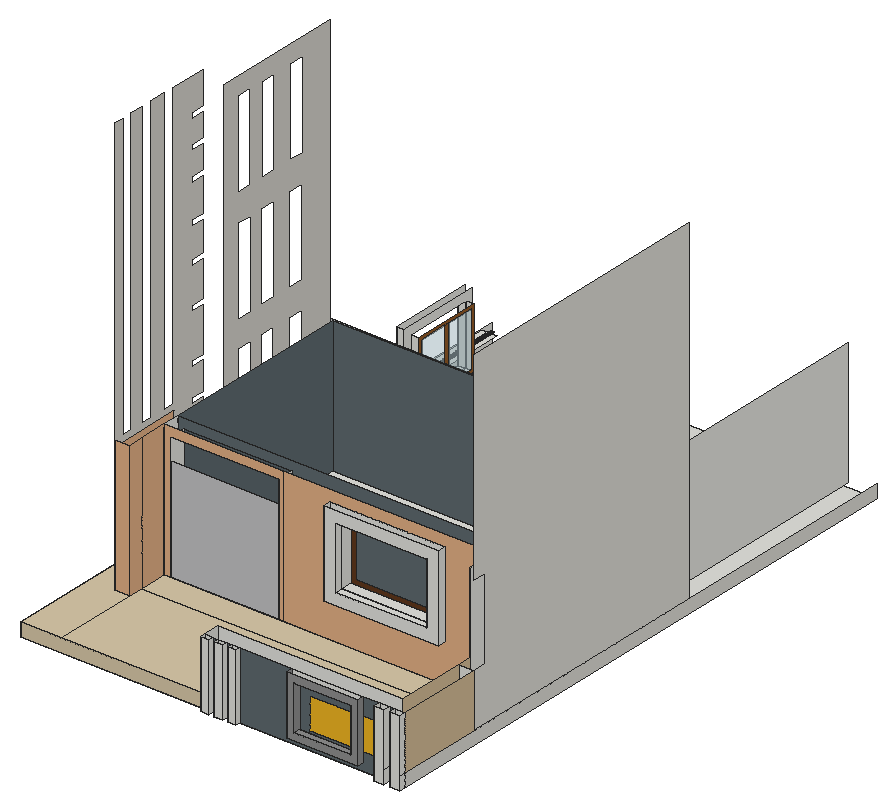
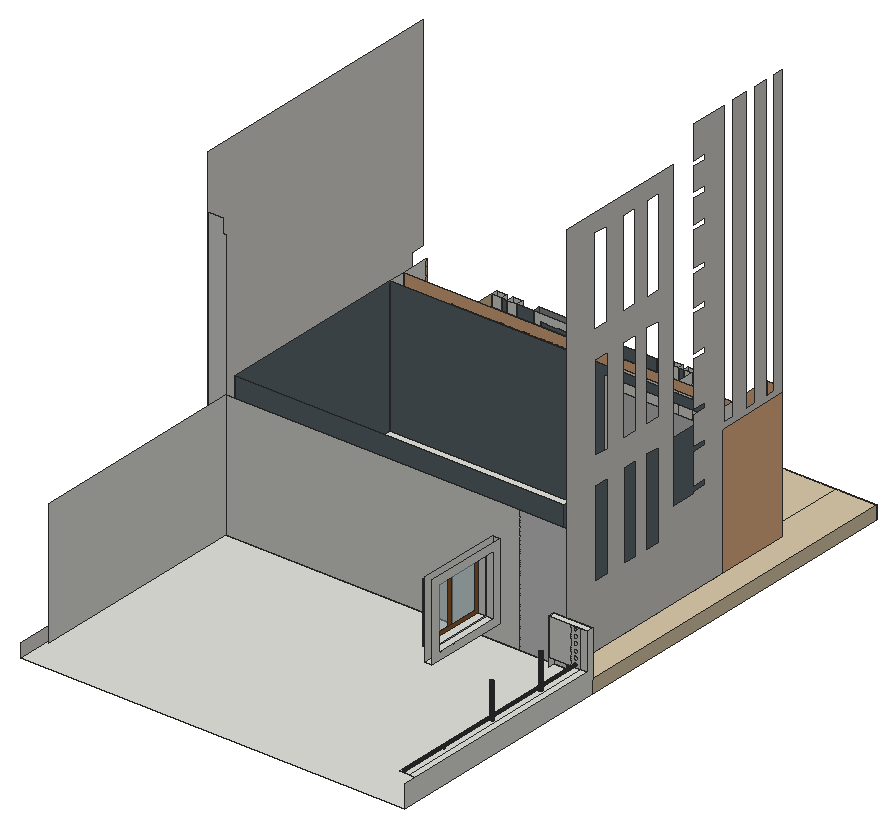
# SketchUp Ruby script. Lengths in inches.
U = 1.inch
M = Sketchup.active_model
def pt(a) = Geom::Point3d.new(a.map { |v| v * U })
def face(e, loops, mat)
  f = e.add_face(loops[0].map { |a| pt(a) })
  loops[1..].each { |l| e.add_face(l.map { |a| pt(a) }).erase! }
  f.material = f.back_material = mat if mat
  f
end
# faces: each face lists its corners as indices into pts; further lists are holes
def faces(e, pts, list, mat = nil) = list.each { |f| face(e, (f[0].is_a?(Array) ? f : [f]).map { |l| l.map { |i| pts[i] } }, mat) }
# xy, xz, yz: faces in a plane at the given z, y or x. An outline is a flat list of corners, or four numbers for a rectangle; further outlines are holes
def ring(l) = l.size == 4 ? [[l[0], l[1]], [l[2], l[1]], [l[2], l[3]], [l[0], l[3]]] : l.each_slice(2).to_a
def flat(e, list, mat, &to3) = list.each { |f| face(e, (f[0].is_a?(Array) ? f : [f]).map { |l| ring(l).map { |u, v| to3.(u, v) } }, mat) }
def xy(e, z, list, mat = nil) = flat(e, list, mat) { |x, y| [x, y, z] }
def xz(e, y, list, mat = nil) = flat(e, list, mat) { |x, z| [x, y, z] }
def yz(e, x, list, mat = nil) = flat(e, list, mat) { |y, z| [x, y, z] }
def lines(e, pts, list) = list.each { |a, b| e.add_line(pt(pts[a]), pt(pts[b])) }
# prism: a flat outline (further loops are holes) pulled along v
def prism(e, loops, v, mat = nil)
  f = face(e, loops, mat); d = Geom::Vector3d.new(v.map { |x| x * U })
  f.pushpull(f.normal.samedirection?(d) ? d.length : -d.length)
end
def box(e, o, s, mat = nil) = prism(e, [[o, [o[0] + s[0], o[1], o[2]], [o[0] + s[0], o[1] + s[1], o[2]], [o[0], o[1] + s[1], o[2]]]], [0, 0, s[2]], mat)
def at(x, y, z, deg = 0) = Geom::Transformation.translation(pt([x, y, z])) * Geom::Transformation.rotation(ORIGIN, Z_AXIS, deg.degrees)
def axes(o, x, y, z) = Geom::Transformation.new([*x, 0, *y, 0, *z, 0, *pt(o).to_a, 1])
def part(name) = M.definitions.add(name)
# library, detail: a bought-in or finely detailed component or shape, given as its bounding box
def library(name, o, s) = part(name).tap { |d| box(d.entities, o, s) }
def detail(e, o, s) = box(e.add_group.entities, o, s)
def put(e, d, t, mat = nil) = e.add_instance(d, t).tap { |i| i.material = mat if mat }
def group(e, t, mat = nil) = e.add_group.tap { |g| g.transformation = t; g.material = mat if mat }.entities
root = M.entities
M.materials.add("[0045_Goldenrod]").color = [239, 181, 35]
M.materials.add("[Blinds Vertical Pattern]").color = [212, 212, 214]
M.materials.add("[Cladding Siding Tan]").color = [226, 176, 133]
M.materials.add("[Color M04]").color = [142, 142, 142]
M.materials.add("[Color M07]").color = [58, 58, 58]
M.materials.add("[Fencing Metal Straight]").color = [194, 195, 196]
M.materials.add("[Field Square Tile]").color = [217, 201, 169]
M.materials.add("[Formica Beige]").color = [211, 187, 149]
M.materials.add("[Formica Speckled Grey]").color = [94, 105, 111]
M.materials.add("[Terrazzo Tile Light]").color = [219, 217, 210]
M.materials.add("[Tile Travertine 2 inch]").color = [211, 208, 201]
M.materials.add("[Translucent Glass Safety]").color = [204, 235, 244]
M.materials["[Translucent Glass Safety]"].alpha = 0.5
M.materials.add("[Wood Floor Parquet]").color = [145, 89, 39]
M.materials.add("[Wood Veneer 01]").color = [96, 56, 29]
xy(root,0,[[499.38,0,512.5625,9.1875],[520.19,0,533.375,9.1875],[265.43,2.6875,276.6,9.1875],[283.37,2.6875,294.54,9.1875],[301.06,2.6875,312.23,9.1875],
  [18.625,9.1875,533.375,797.6875]])
xy(root,10.4375,[[382.41,0,477.59,9.1875]],"[Color M04]")
xy(root,18,[[53.375,123.625,53.375,483.625,533.375,483.625,533.375,123.625,513.45,123.625,513.45,463.7,73.3,463.7,73.3,123.625],[73.3,181.59,81.47,204.11],[81.47,181.59,226.34,204.11],[226.34,181.59,513.45,204.11],[73.3,204.11,513.45,463.7]])
xy(root,18,[[18.625,9.1875,73.3,9.1875,73.3,123.625,53.375,123.625,53.375,483.625,18.625,483.625],[73.3,9.1875,265.43,9.1875,265.43,31.125,513.45,31.125,513.45,143.55,73.3,143.55],[73.3,143.55,513.45,181.59]],"[Field Square Tile]")
xy(root,20.19,[[392.16,0,467.84,9.1875]],"[Color M04]")
xy(root,29.4375,[[18.625,492.63,26.76,779.875],[[26.76,492.63,40.07,779.875],[32.79,632.33,32.19,632.41,31.63,632.64,31.15,633.01,30.79,633.49,30.56,634.04,30.48,634.64,30.56,635.24,30.79,635.8,31.15,636.28,31.63,636.65,32.19,636.875,32.79,636.96,33.39,636.875,33.95,636.65,34.42,636.28,34.79,635.8,35.02,635.24,35.1,634.64,35.02,634.04,34.79,633.49,34.42,633.01,33.95,632.64,33.39,632.41],[32.79,550.08,32.19,550.16,31.63,550.39,31.15,550.76,30.79,551.24,30.56,551.79,30.48,552.39,30.56,552.99,30.79,553.55,31.15,554.03,31.63,554.4,32.19,554.625,32.79,554.71,33.39,554.625,33.95,554.4,34.42,554.03,34.79,553.55,35.02,552.99,35.1,552.39,35.02,551.79,34.79,551.24,34.42,550.76,33.95,550.39,33.39,550.16],[32.79,711.89,32.19,711.97,31.63,712.2,31.15,712.57,30.79,713.05,30.56,713.61,30.48,714.21,30.56,714.8,30.79,715.36,31.15,715.84,31.63,716.21,32.19,716.4375,32.79,716.52,33.39,716.4375,33.95,716.21,34.42,715.84,34.79,715.36,35.02,714.8,35.1,714.21,35.02,713.61,34.79,713.05,34.42,712.57,33.95,712.2,33.39,711.97]],[32.79,550.08,32.19,550.16,31.63,550.39,31.15,550.76,30.79,551.24,30.56,551.79,30.48,552.39,30.56,552.99,30.79,553.55,31.15,554.03,31.63,554.4,32.19,554.625,32.79,554.71,33.39,554.625,33.95,554.4,34.42,554.03,34.79,553.55,35.02,552.99,35.1,552.39,35.02,551.79,34.79,551.24,34.42,550.76,33.95,550.39,33.39,550.16],[32.79,632.33,32.19,632.41,31.63,632.64,31.15,633.01,30.79,633.49,30.56,634.04,30.48,634.64,30.56,635.24,30.79,635.8,31.15,636.28,31.63,636.65,32.19,636.875,32.79,636.96,33.39,636.875,33.95,636.65,34.42,636.28,34.79,635.8,35.02,635.24,35.1,634.64,35.02,634.04,34.79,633.49,34.42,633.01,33.95,632.64,33.39,632.41]])
xy(root,68.97,[[295.4375,171.21,449,181.59]])
xy(root,72.6,[[106.94,528.53,116.75,641.54]])
xy(root,75.3125,[[32.79,550.08,33.39,550.16,33.95,550.39,34.42,550.76,34.79,551.24,35.02,551.79,35.1,552.39,35.02,552.99,34.79,553.55,34.42,554.03,33.95,554.4,33.39,554.625,32.79,554.71,32.19,554.625,31.63,554.4,31.15,554.03,30.79,553.55,30.56,552.99,30.48,552.39,30.56,551.79,30.79,551.24,31.15,550.76,31.63,550.39,32.19,550.16]],"[Color M07]")
xy(root,76.375,[[32.79,632.33,33.39,632.41,33.95,632.64,34.42,633.01,34.79,633.49,35.02,634.04,35.1,634.64,35.02,635.24,34.79,635.8,34.42,636.28,33.95,636.65,33.39,636.875,32.79,636.96,32.19,636.875,31.63,636.65,31.15,636.28,30.79,635.8,30.56,635.24,30.48,634.64,30.56,634.04,30.79,633.49,31.15,633.01,31.63,632.64,32.19,632.41]],"[Color M07]")
xy(root,78.6875,[[18.625,483.625,70.21,492.63]])
xy(root,79.81,[[392.16,0,467.84,9.1875]])
xy(root,83.1,[[106.94,539.02,116.75,631.05],[116.75,539.02,128.38,631.05]])
xy(root,84.57,[[311.03,171.21,433.4,181.59],[311.03,181.59,433.4,197.15]])
xz(root,0,[[499.38,0,512.5625,89.5625],[520.19,0,533.375,89.5625]])
xz(root,0,[[[382.41,10.4375,477.59,89.5625],[392.16,20.19,467.84,79.81]]],"[Color M04]")
xz(root,2.6875,[[265.43,0,276.6,89.5625],[283.37,0,294.54,89.5625],[301.06,0,312.23,89.5625]])
xz(root,9.1875,[[265.43,0,276.6,89.5625],[283.37,0,294.54,89.5625],[301.06,0,312.23,89.5625],[499.38,0,512.5625,89.5625],[520.19,0,533.375,89.5625],
  [[382.41,10.4375,477.59,89.5625],[392.16,20.19,467.84,79.81]]])
xz(root,9.1875,[[406.65,23.29,467.84,65.73],[477.59,23.29,499.38,65.73]],"[0045_Goldenrod]")
xz(root,9.1875,[[18.625,0,265.43,18]],"[Field Square Tile]")
xz(root,9.1875,[[276.6,0,283.37,89.5625],[294.54,0,301.06,89.5625],[312.23,0,499.38,0,499.38,23.29,477.59,23.29,477.59,10.4375,382.41,10.4375,382.41,89.5625,312.23,89.5625],[512.5625,0,520.19,89.5625],[392.16,20.19,467.84,20.19,467.84,23.29,406.65,23.29,406.65,65.73,467.84,65.73,467.84,79.81,392.16,79.81],
  [477.59,65.73,499.38,89.5625]],"[Formica Speckled Grey]")
xz(root,31.125,[[265.43,18,513.45,89.5625]])
xz(root,123.625,[[513.45,18,533.375,89.5625]])
xz(root,123.625,[[53.375,18,73.3,198]],"[Cladding Siding Tan]")
xz(root,171.21,[[[295.4375,68.97,449,183.35],[311.03,84.57,433.4,167.75]]])
xz(root,181.59,[[[295.4375,68.97,449,183.35],[311.03,84.57,433.4,167.75]]])
xz(root,181.59,[[73.3,18,81.47,18,81.47,186,226.34,186,226.34,18,231.56,18,231.56,198,73.3,198],[[231.56,18,513.45,198],[295.4375,68.97,449,183.35]]],"[Cladding Siding Tan]")
xz(root,181.59,[[81.47,18,226.34,156.98]],"[Fencing Metal Straight]")
xz(root,197.15,[[[311.03,84.57,433.4,167.75],[316.66,90.2,427.78,162.125]]],"[Wood Veneer 01]")
xz(root,204.11,[[73.3,18,73.3,198,513.45,198,513.45,18,226.34,18,226.34,186,81.47,186,81.47,18]],"[Formica Speckled Grey]")
xz(root,463.7,[[73.3,18,513.45,198]],"[Formica Speckled Grey]")
xz(root,483.625,[[18.625,18,53.375,78.6875],[53.375,18,70.21,78.6875],[116.75,18,509.21,185.6875],[509.21,18,509.21,378,513.45,378,513.45,396.875,533.375,396.875,533.375,18]])
xz(root,483.625,[[70.21,18,70.21,78.6875,53.375,78.6875,53.375,185.6875,116.75,185.6875,116.75,18]],"[Blinds Vertical Pattern]")
xz(root,492.63,[[18.625,29.4375,26.76,78.6875],[[26.76,29.4375,40.07,78.6875],[34.16,73.8,34.63,73.87,35.07,74.05,35.44,74.34,35.73,74.71,35.91,75.15,35.97,75.62,35.91,76.09,35.73,76.52,35.44,76.9,35.07,77.1875,34.63,77.37,34.16,77.43,33.69,77.37,33.25,77.1875,32.88,76.9,32.59,76.52,32.41,76.09,32.35,75.62,32.41,75.15,32.59,74.71,32.88,74.34,33.25,74.05,33.69,73.87],[34.16,39.43,34.63,39.49,35.07,39.67,35.44,39.96,35.73,40.34,35.91,40.77,35.97,41.24,35.91,41.71,35.73,42.15,35.44,42.52,35.07,42.8125,34.63,42.99,34.16,43.05,33.69,42.99,33.25,42.8125,32.88,42.52,32.59,42.15,32.41,41.71,32.35,41.24,32.41,40.77,32.59,40.34,32.88,39.96,33.25,39.67,33.69,39.49],[34.16,65.12,34.63,65.18,35.07,65.36,35.44,65.65,35.73,66.02,35.91,66.46,35.97,66.93,35.91,67.4,35.73,67.84,35.44,68.21,35.07,68.5,34.63,68.68,34.16,68.74,33.69,68.68,33.25,68.5,32.88,68.21,32.59,67.84,32.41,67.4,32.35,66.93,32.41,66.46,32.59,66.02,32.88,65.65,33.25,65.36,33.69,65.18],[34.16,47.68,34.63,47.74,35.07,47.92,35.44,48.21,35.73,48.59,35.91,49.02,35.97,49.49,35.91,49.96,35.73,50.4,35.44,50.77,35.07,51.0625,34.63,51.24,34.16,51.3,33.69,51.24,33.25,51.0625,32.88,50.77,32.59,50.4,32.41,49.96,32.35,49.49,32.41,49.02,32.59,48.59,32.88,48.21,33.25,47.92,33.69,47.74],[34.16,56.74,34.63,56.8,35.07,56.99,35.44,57.27,35.73,57.65,35.91,58.09,35.97,58.55,35.91,59.02,35.73,59.46,35.44,59.84,35.07,60.125,34.63,60.31,34.16,60.37,33.69,60.31,33.25,60.125,32.88,59.84,32.59,59.46,32.41,59.02,32.35,58.55,32.41,58.09,32.59,57.65,32.88,57.27,33.25,56.99,33.69,56.8],[34.16,31.24,34.63,31.3,35.07,31.49,35.44,31.77,35.73,32.15,35.91,32.59,35.97,33.05,35.91,33.52,35.73,33.96,35.44,34.34,35.07,34.625,34.63,34.81,34.16,34.87,33.69,34.81,33.25,34.625,32.88,34.34,32.59,33.96,32.41,33.52,32.35,33.05,32.41,32.59,32.59,32.15,32.88,31.77,33.25,31.49,33.69,31.3]],[40.07,29.4375,70.21,78.6875],[34.16,31.24,34.63,31.3,35.07,31.49,35.44,31.77,35.73,32.15,35.91,32.59,35.97,33.05,35.91,33.52,35.73,33.96,35.44,34.34,35.07,34.625,34.63,34.81,34.16,34.87,33.69,34.81,33.25,34.625,32.88,34.34,32.59,33.96,32.41,33.52,32.35,33.05,32.41,32.59,32.59,32.15,32.88,31.77,33.25,31.49,33.69,31.3],[34.16,39.43,34.63,39.49,35.07,39.67,35.44,39.96,35.73,40.34,35.91,40.77,35.97,41.24,35.91,41.71,35.73,42.15,35.44,42.52,35.07,42.8125,34.63,42.99,34.16,43.05,33.69,42.99,33.25,42.8125,32.88,42.52,32.59,42.15,32.41,41.71,32.35,41.24,32.41,40.77,32.59,40.34,32.88,39.96,33.25,39.67,33.69,39.49],
  [34.16,47.68,34.63,47.74,35.07,47.92,35.44,48.21,35.73,48.59,35.91,49.02,35.97,49.49,35.91,49.96,35.73,50.4,35.44,50.77,35.07,51.0625,34.63,51.24,34.16,51.3,33.69,51.24,33.25,51.0625,32.88,50.77,32.59,50.4,32.41,49.96,32.35,49.49,32.41,49.02,32.59,48.59,32.88,48.21,33.25,47.92,33.69,47.74],[34.16,56.74,34.63,56.8,35.07,56.99,35.44,57.27,35.73,57.65,35.91,58.09,35.97,58.55,35.91,59.02,35.73,59.46,35.44,59.84,35.07,60.125,34.63,60.31,34.16,60.37,33.69,60.31,33.25,60.125,32.88,59.84,32.59,59.46,32.41,59.02,32.35,58.55,32.41,58.09,32.59,57.65,32.88,57.27,33.25,56.99,33.69,56.8],[34.16,65.12,34.63,65.18,35.07,65.36,35.44,65.65,35.73,66.02,35.91,66.46,35.97,66.93,35.91,67.4,35.73,67.84,35.44,68.21,35.07,68.5,34.63,68.68,34.16,68.74,33.69,68.68,33.25,68.5,32.88,68.21,32.59,67.84,32.41,67.4,32.35,66.93,32.41,66.46,32.59,66.02,32.88,65.65,33.25,65.36,33.69,65.18],[34.16,73.8,34.63,73.87,35.07,74.05,35.44,74.34,35.73,74.71,35.91,75.15,35.97,75.62,35.91,76.09,35.73,76.52,35.44,76.9,35.07,77.1875,34.63,77.37,34.16,77.43,33.69,77.37,33.25,77.1875,32.88,76.9,32.59,76.52,32.41,76.09,32.35,75.62,32.41,75.15,32.59,74.71,32.88,74.34,33.25,74.05,33.69,73.87]])
xz(root,528.53,[[106.94,72.6,116.75,174.66]])
xz(root,539.02,[[106.94,83.1,116.75,164.17],[116.75,83.1,128.38,164.17]])
xz(root,631.05,[[106.94,83.1,116.75,164.17],[116.75,83.1,128.38,164.17]])
yz(root,18.625,[[483.625,0,483.625,78.6875,492.63,78.6875,492.63,29.4375,797.6875,29.4375,797.6875,0]])
yz(root,18.625,[[9.1875,0,483.625,18]],"[Field Square Tile]")
yz(root,53.375,[[123.625,18,222.87,189.9375]],"[Cladding Siding Tan]")
yz(root,53.375,[[[222.87,18,222.87,189.9375,123.625,189.9375,123.625,577.3125,136.75,577.3125,136.75,198,151.32,198,151.32,577.3125,169.81,577.3125,169.81,198,184.38,198,184.38,577.3125,206.12,577.3125,206.12,198,220.7,198,220.7,577.3125,270.46,577.3125,270.46,533.22,253.03,533.22,253.03,526.41,270.46,526.41,270.46,495.16,253.03,495.16,253.03,488.34,270.46,488.34,270.46,456.47,253.03,456.47,253.03,449.66,270.46,449.66,270.46,404.47,253.03,404.47,253.03,397.66,270.46,397.66,270.46,356.97,253.03,356.97,253.03,350.16,270.46,350.16,270.46,301.97,253.03,301.97,253.03,295.16,270.46,295.16,270.46,235.53,253.03,235.53,253.03,228.72,270.46,228.72,270.46,191.16,253.03,191.16,253.03,184.34,270.46,184.34,270.46,143.41,253.03,143.41,253.03,136.59,270.46,136.59,270.46,134.2,306.125,134.2,306.125,543.2,483.625,543.2,483.625,18],[417,404.29,438.25,519.67],[415.62,251.86,436.87,367.23],[415.12,101.04,436.37,216.42],[369.37,404.29,390.62,519.67],[329.18,404.29,350.43,519.67],[368.62,251.86,389.87,367.23],[329.31,251.86,350.56,367.23],[367.37,101.04,388.62,216.42],[329.87,101.04,351.12,216.42]]],"[Tile Travertine 2 inch]")
yz(root,70.21,[[483.625,18,492.63,78.6875]])
yz(root,73.3,[[181.59,18,204.11,198]])
yz(root,73.3,[[123.625,18,143.55,198],[143.55,18,181.59,198]],"[Cladding Siding Tan]")
yz(root,73.3,[[204.11,18,463.7,198]],"[Formica Speckled Grey]")
yz(root,81.47,[[181.59,18,204.11,186]])
yz(root,106.94,[[[528.53,72.6,641.54,174.66],[539.02,83.1,631.05,164.17]]])
yz(root,116.75,[[[528.53,72.6,641.54,174.66],[539.02,83.1,631.05,164.17]]])
yz(root,128.38,[[543,87.08,582.62,160.19],[588.03,87.08,627.07,160.19]],"[Translucent Glass Safety]")
yz(root,128.38,[[[539.02,83.1,631.05,164.17],[543,87.08,627.07,160.19]],[582.62,87.08,588.03,160.19]],"[Wood Floor Parquet]")
yz(root,226.34,[[181.59,18,204.11,186]])
yz(root,265.43,[[2.6875,0,9.1875,18],[2.6875,18,9.1875,89.5625],[9.1875,18,31.125,89.5625]])
yz(root,276.6,[[2.6875,0,9.1875,89.5625]])
yz(root,283.37,[[2.6875,0,9.1875,18],[2.6875,18,9.1875,89.5625]])
yz(root,294.54,[[2.6875,0,9.1875,89.5625]])
yz(root,295.4375,[[171.21,68.97,181.59,183.35]])
yz(root,301.06,[[2.6875,0,9.1875,18],[2.6875,18,9.1875,89.5625]])
yz(root,311.03,[[171.21,84.57,181.59,167.75],[181.59,84.57,197.15,167.75]])
yz(root,312.23,[[2.6875,0,9.1875,89.5625]])
yz(root,382.41,[[0,10.4375,9.1875,89.5625]],"[Color M04]")
yz(root,392.16,[[0,20.19,9.1875,79.81]],"[Color M04]")
yz(root,433.4,[[171.21,84.57,181.59,167.75],[181.59,84.57,197.15,167.75]])
yz(root,449,[[171.21,68.97,181.59,183.35]])
yz(root,467.84,[[0,20.19,9.1875,23.29],[0,23.29,9.1875,65.73],[0,65.73,9.1875,79.81]],"[Color M04]")
yz(root,477.59,[[0,10.4375,9.1875,89.5625]],"[Color M04]")
yz(root,499.38,[[0,0,9.1875,89.5625]])
yz(root,509.21,[[483.625,18,779.875,185.6875]])
yz(root,512.5625,[[0,0,9.1875,18],[0,18,9.1875,89.5625]])
yz(root,513.45,[[143.55,18,181.59,198],[181.59,18,204.11,198]])
yz(root,513.45,[[31.125,18,123.625,89.5625],[123.625,18,123.625,89.5625,142.4375,89.5625,142.4375,198,143.55,198,143.55,18]],"[Formica Beige]")
yz(root,513.45,[[204.11,18,463.7,198]],"[Formica Speckled Grey]")
yz(root,520.19,[[0,0,9.1875,89.5625]])
yz(root,533.375,[[0,0,9.1875,18],[0,18,9.1875,89.5625]])
yz(root,533.375,[[9.1875,18,123.625,89.5625]],"[Formica Beige]")
yz(root,533.375,[[9.1875,0,797.6875,18],[123.625,18,483.625,18,483.625,468.5,123.625,468.5,123.625,198,142.4375,198,142.4375,89.5625,123.625,89.5625]],"[Terrazzo Tile Light]")
p = [[32.19,550.16,29.4375],[32.79,550.08,29.4375],[32.79,550.08,75.3125],[32.19,550.16,75.3125],[33.39,550.16,29.4375],[33.39,550.16,75.3125],
  [31.63,550.39,29.4375],[31.63,550.39,75.3125],[33.95,550.39,29.4375],[33.95,550.39,75.3125],[31.15,550.76,29.4375],[31.15,550.76,75.3125],
  [34.42,550.76,29.4375],[34.42,550.76,75.3125],[30.79,551.24,29.4375],[30.79,551.24,75.3125],[34.79,551.24,29.4375],[34.79,551.24,75.3125],
  [30.56,551.79,29.4375],[30.56,551.79,75.3125],[35.02,551.79,29.4375],[35.02,551.79,75.3125],[30.48,552.39,29.4375],[30.48,552.39,75.3125],
  [35.1,552.39,29.4375],[35.1,552.39,75.3125],[30.56,552.99,29.4375],[30.56,552.99,75.3125],[35.02,552.99,29.4375],[35.02,552.99,75.3125],
  [30.79,553.55,29.4375],[30.79,553.55,75.3125],[34.79,553.55,29.4375],[34.79,553.55,75.3125],[31.15,554.03,29.4375],[31.15,554.03,75.3125],
  [34.42,554.03,29.4375],[34.42,554.03,75.3125],[31.63,554.4,29.4375],[31.63,554.4,75.3125],[33.95,554.4,29.4375],[33.95,554.4,75.3125],
  [32.19,554.625,29.4375],[32.19,554.625,75.3125],[33.39,554.625,29.4375],[33.39,554.625,75.3125],[32.79,554.71,29.4375],[32.79,554.71,75.3125],
  [32.19,632.41,29.4375],[32.79,632.33,29.4375],[32.79,632.33,76.375],[32.19,632.41,76.375],[33.39,632.41,29.4375],[33.39,632.41,76.375],
  [31.63,632.64,29.4375],[31.63,632.64,76.375],[33.95,632.64,29.4375],[33.95,632.64,76.375],[31.15,633.01,29.4375],[31.15,633.01,76.375],
  [34.42,633.01,29.4375],[34.42,633.01,76.375],[30.79,633.49,29.4375],[30.79,633.49,76.375],[34.79,633.49,29.4375],[34.79,633.49,76.375],
  [30.56,634.04,29.4375],[30.56,634.04,76.375],[35.02,634.04,29.4375],[35.02,634.04,76.375],[30.48,634.64,29.4375],[30.48,634.64,76.375],
  [35.1,634.64,29.4375],[35.1,634.64,76.375],[30.56,635.24,29.4375],[30.56,635.24,76.375],[35.02,635.24,29.4375],[35.02,635.24,76.375],
  [30.79,635.8,29.4375],[30.79,635.8,76.375],[34.79,635.8,29.4375],[34.79,635.8,76.375],[31.15,636.28,29.4375],[31.15,636.28,76.375],
  [34.42,636.28,29.4375],[34.42,636.28,76.375],[34.16,492.63,31.24],[33.69,492.63,31.3],[33.69,779.875,31.3],[34.16,779.875,31.24],
  [34.63,492.63,31.3],[34.63,779.875,31.3],[33.25,492.63,31.49],[33.25,779.875,31.49],[35.07,492.63,31.49],[35.07,779.875,31.49],
  [32.88,492.63,31.77],[32.88,779.875,31.77],[35.44,492.63,31.77],[35.44,779.875,31.77],[32.59,492.63,32.15],[32.59,779.875,32.15],
  [35.73,492.63,32.15],[35.73,779.875,32.15],[32.41,492.63,32.59],[32.41,779.875,32.59],[35.91,492.63,32.59],[35.91,779.875,32.59],
  [32.35,492.63,33.05],[32.35,779.875,33.05],[35.97,492.63,33.05],[35.97,779.875,33.05],[32.41,492.63,33.52],[32.41,779.875,33.52],
  [35.91,492.63,33.52],[35.91,779.875,33.52],[513.45,31.125,18],[513.45,9.1875,18]]
faces(root,p,[[0,1,2,3],[1,4,5,2],[6,0,3,7],[4,8,9,5],[10,6,7,11],[8,12,13,9],[14,10,11,15],[12,16,17,13],
  [18,14,15,19],[16,20,21,17],[22,18,19,23],[20,24,25,21],[26,22,23,27],[24,28,29,25],[30,26,27,31],[28,32,33,29],
  [34,30,31,35],[32,36,37,33],[38,34,35,39],[36,40,41,37],[42,38,39,43],[40,44,45,41],[46,42,43,47],[44,46,47,45],
  [48,49,50,51],[49,52,53,50],[54,48,51,55],[52,56,57,53],[58,54,55,59],[56,60,61,57],[62,58,59,63],[60,64,65,61],
  [66,62,63,67],[64,68,69,65],[70,66,67,71],[68,72,73,69],[74,70,71,75],[72,76,77,73],[78,74,75,79],[76,80,81,77],
  [82,78,79,83],[80,84,85,81],[86,87,88,89],[90,86,89,91],[87,92,93,88],[94,90,91,95],[92,96,97,93],[98,94,95,99],
  [96,100,101,97],[102,98,99,103],[100,104,105,101],[106,102,103,107],[104,108,109,105],[110,106,107,111],[108,112,113,109],[114,110,111,115]],"[Color M07]")
lines(root,p,[[116,117]])
